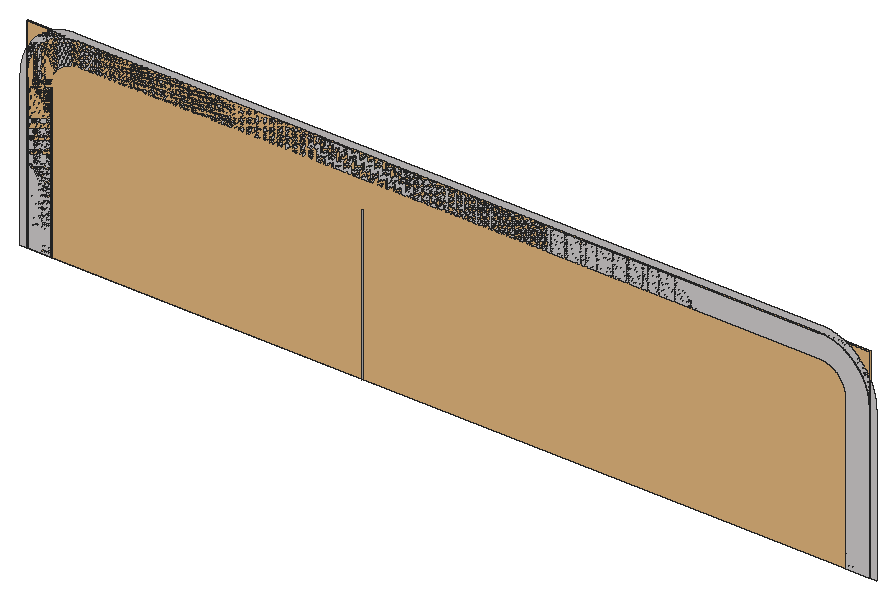
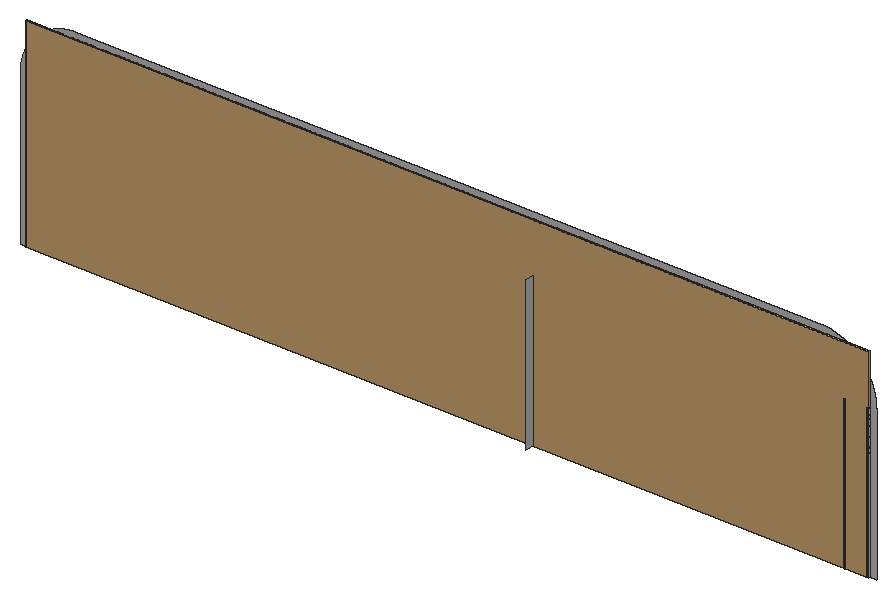
# SketchUp Ruby script. Lengths in inches.
U = 1.inch
M = Sketchup.active_model
def pt(a) = Geom::Point3d.new(a.map { |v| v * U })
def face(e, loops, mat)
  f = e.add_face(loops[0].map { |a| pt(a) })
  loops[1..].each { |l| e.add_face(l.map { |a| pt(a) }).erase! }
  f.material = f.back_material = mat if mat
  f
end
# faces: each face lists its corners as indices into pts; further lists are holes
def faces(e, pts, list, mat = nil) = list.each { |f| face(e, (f[0].is_a?(Array) ? f : [f]).map { |l| l.map { |i| pts[i] } }, mat) }
# xy, xz, yz: faces in a plane at the given z, y or x. An outline is a flat list of corners, or four numbers for a rectangle; further outlines are holes
def ring(l) = l.size == 4 ? [[l[0], l[1]], [l[2], l[1]], [l[2], l[3]], [l[0], l[3]]] : l.each_slice(2).to_a
def flat(e, list, mat, &to3) = list.each { |f| face(e, (f[0].is_a?(Array) ? f : [f]).map { |l| ring(l).map { |u, v| to3.(u, v) } }, mat) }
def xy(e, z, list, mat = nil) = flat(e, list, mat) { |x, y| [x, y, z] }
def xz(e, y, list, mat = nil) = flat(e, list, mat) { |x, z| [x, y, z] }
def yz(e, x, list, mat = nil) = flat(e, list, mat) { |y, z| [x, y, z] }
def lines(e, pts, list) = list.each { |a, b| e.add_line(pt(pts[a]), pt(pts[b])) }
# prism: a flat outline (further loops are holes) pulled along v
def prism(e, loops, v, mat = nil)
  f = face(e, loops, mat); d = Geom::Vector3d.new(v.map { |x| x * U })
  f.pushpull(f.normal.samedirection?(d) ? d.length : -d.length)
end
def box(e, o, s, mat = nil) = prism(e, [[o, [o[0] + s[0], o[1], o[2]], [o[0] + s[0], o[1] + s[1], o[2]], [o[0], o[1] + s[1], o[2]]]], [0, 0, s[2]], mat)
def at(x, y, z, deg = 0) = Geom::Transformation.translation(pt([x, y, z])) * Geom::Transformation.rotation(ORIGIN, Z_AXIS, deg.degrees)
def axes(o, x, y, z) = Geom::Transformation.new([*x, 0, *y, 0, *z, 0, *pt(o).to_a, 1])
def part(name) = M.definitions.add(name)
# library, detail: a bought-in or finely detailed component or shape, given as its bounding box
def library(name, o, s) = part(name).tap { |d| box(d.entities, o, s) }
def detail(e, o, s) = box(e.add_group.entities, o, s)
def put(e, d, t, mat = nil) = e.add_instance(d, t).tap { |i| i.material = mat if mat }
def group(e, t, mat = nil) = e.add_group.tap { |g| g.transformation = t; g.material = mat if mat }.entities
root = M.entities
M.materials.add("Outer Light - 1").color = [251, 216, 141]
M.materials.add("[Quartz Light Brown]").color = [215, 212, 212]
M.materials.add("[Stone Sandstone Ashlar Light]").color = [201, 199, 196]
c1 = library("Group\#55",[0,0,0],[532,1,128])
xz(root,38,[[0,-12,4,-12,4,84.5,4.01,84.75,4.02,85.01,4.02,85.26,4.04,85.51,4.05,85.76,4.0625,86.01,4.08,86.26,4.14,87.01,4.17,87.26,4.19,87.51,4.28,88.26,4.36,88.76,4.39,89.01,4.43,89.25,4.48,89.5,4.52,89.75,4.57,90,4.61,90.24,4.66,90.49,4.72,90.74,4.77,90.98,4.83,91.23,4.88,91.47,4.94,91.71,5.01,91.96,5.13,92.44,5.2,92.6875,5.27,92.93,5.41,93.41,5.57,93.89,5.64,94.13,5.73,94.37,5.81,94.6,5.89,94.84,5.98,95.08,6.07,95.3125,6.16,95.55,6.34,96.01,6.4375,96.25,6.53,96.48,6.63,96.71,6.73,96.9375,6.84,97.17,6.9375,97.4,7.05,97.625,7.15,97.85,7.26,98.08,7.375,98.3,7.6,98.75,7.72,98.97,7.84,99.2,8.08,99.64,8.2,99.85,8.59,100.51,8.85,100.93,8.98,101.15,9.12,101.36,9.25,101.57,9.53,101.99,9.68,102.19,9.96,102.61,10.41,103.21,10.5625,103.41,10.72,103.61,10.87,103.8125,11.03,104.01,11.18,104.2,11.34,104.4,11.5,104.59,11.67,104.78,11.83,104.97,12,105.16,12.16,105.35,12.33,105.54,12.5,105.72,12.67,105.91,12.85,106.09,13.02,106.27,13.2,106.45,13.37,106.63,13.55,106.8,13.73,106.98,13.91,107.15,14.09,107.33,14.28,107.5,14.46,107.67,14.65,107.84,14.84,108,15.03,108.17,15.22,108.33,15.41,108.5,15.6,108.66,15.8,108.82,15.99,108.97,16.1875,109.13,16.39,109.28,16.59,109.4375,16.79,109.59,17.39,110.04,17.81,110.32,18.01,110.47,18.43,110.75,18.64,110.88,18.85,111.02,19.07,111.15,19.49,111.41,20.15,111.8,20.36,111.92,20.8,112.16,21.03,112.28,21.25,112.4,21.7,112.625,21.92,112.74,22.15,112.85,22.375,112.95,22.6,113.0625,22.83,113.16,23.0625,113.27,23.29,113.37,23.52,113.47,23.75,113.5625,23.99,113.66,24.45,113.84,24.6875,113.93,24.92,114.02,25.16,114.11,25.4,114.19,25.63,114.27,25.87,114.36,26.11,114.43,26.59,114.59,27.07,114.73,27.3125,114.8,27.56,114.87,28.04,114.99,28.29,115.06,28.53,115.12,28.77,115.17,29.02,115.23,29.26,115.28,29.51,115.34,29.76,115.39,30,115.43,30.25,115.48,30.5,115.52,30.75,115.57,30.99,115.61,31.24,115.64,31.74,115.72,32.49,115.81,32.74,115.83,32.99,115.86,33.74,115.92,33.99,115.9375,34.24,115.95,34.49,115.96,34.74,115.98,34.99,115.98,35.25,115.99,35.5,116,504.5,116,504.75,115.99,505.01,115.98,505.26,115.98,505.51,115.96,505.76,115.95,506.01,115.9375,506.26,115.92,507.01,115.86,507.26,115.83,507.51,115.81,508.26,115.72,508.76,115.64,509.01,115.61,509.25,115.57,509.5,115.52,509.75,115.48,510,115.43,510.24,115.39,510.49,115.34,510.74,115.28,510.98,115.23,511.23,115.17,511.47,115.12,511.71,115.06,511.96,114.99,512.44,114.87,512.6875,114.8,512.93,114.73,513.41,114.59,513.89,114.43,514.13,114.36,514.37,114.27,514.6,114.19,514.84,114.11,515.08,114.02,515.3125,113.93,515.55,113.84,516.01,113.66,516.25,113.5625,516.48,113.47,516.71,113.37,516.9375,113.27,517.17,113.16,517.4,113.0625,517.625,112.95,517.85,112.85,518.08,112.74,518.3,112.625,518.75,112.4,518.97,112.28,519.2,112.16,519.64,111.92,519.85,111.8,520.51,111.41,520.93,111.15,521.15,111.02,521.36,110.88,521.57,110.75,521.99,110.47,522.19,110.32,522.61,110.04,523.21,109.59,523.41,109.4375,523.61,109.28,523.8125,109.13,524.01,108.97,524.2,108.82,524.4,108.66,524.59,108.5,524.78,108.33,524.97,108.17,525.16,108,525.35,107.84,525.54,107.67,525.72,107.5,525.91,107.33,526.09,107.15,526.27,106.98,526.45,106.8,526.63,106.63,526.8,106.45,526.98,106.27,527.15,106.09,527.33,105.91,527.5,105.72,527.67,105.54,527.84,105.35,528,105.16,528.17,104.97,528.33,104.78,528.5,104.59,528.66,104.4,528.82,104.2,528.97,104.01,529.13,103.8125,529.28,103.61,529.4375,103.41,529.59,103.21,530.04,102.61,530.32,102.19,530.47,101.99,530.75,101.57,530.88,101.36,531.02,101.15,531.15,100.93,531.41,100.51,531.8,99.85,531.92,99.64,532.16,99.2,532.28,98.97,532.4,98.75,532.625,98.3,532.74,98.08,532.85,97.85,532.95,97.625,533.0625,97.4,533.16,97.17,533.27,96.9375,533.37,96.71,533.47,96.48,533.5625,96.25,533.66,96.01,533.84,95.55,533.93,95.3125,534.02,95.08,534.11,94.84,534.19,94.6,534.27,94.37,534.36,94.13,534.43,93.89,534.59,93.41,534.73,92.93,534.8,92.6875,534.87,92.44,534.99,91.96,535.06,91.71,535.12,91.47,535.17,91.23,535.23,90.98,535.28,90.74,535.34,90.49,535.39,90.24,535.43,90,535.48,89.75,535.52,89.5,535.57,89.25,535.61,89.01,535.64,88.76,535.72,88.26,535.81,87.51,535.83,87.26,535.86,87.01,535.92,86.26,535.9375,86.01,535.95,85.76,535.96,85.51,535.98,85.26,535.98,85.01,535.99,84.75,536,84.5,536,-12,540,-12,540,84.57,539.97,85.41,539.96,85.7,539.95,85.98,539.89,86.82,539.87,87.11,539.84,87.39,539.8125,87.67,539.78,87.95,539.72,88.51,539.56,89.63,539.51,89.91,539.46,90.1875,539.41,90.47,539.36,90.75,539.31,91.02,539.19,91.58,539.13,91.85,539.07,92.13,539.01,92.4,538.9375,92.68,538.8,93.23,538.72,93.5,538.65,93.77,538.49,94.31,538.41,94.59,538.32,94.86,538.24,95.125,538.15,95.39,537.97,95.93,537.87,96.19,537.77,96.46,537.68,96.73,537.58,96.99,537.47,97.25,537.37,97.51,537.26,97.78,536.93,98.56,536.8125,98.81,536.69,99.07,536.57,99.33,536.45,99.58,536.33,99.84,536.2,100.09,536.08,100.34,535.95,100.6,535.82,100.85,535.68,101.09,535.55,101.34,535.27,101.84,535.13,102.08,534.99,102.33,534.84,102.57,534.7,102.81,534.4,103.29,534.24,103.53,534.09,103.76,533.77,104.24,533.62,104.47,533.45,104.7,533.29,104.93,532.96,105.39,532.79,105.62,532.45,106.06,532.27,106.29,532.1,106.51,531.74,106.95,531.56,107.16,531.375,107.38,531.19,107.59,531,107.81,530.82,108.02,530.625,108.23,530.4375,108.4375,530.24,108.64,530.05,108.85,529.85,109.05,529.65,109.26,529.46,109.46,529.26,109.65,529.05,109.85,528.85,110.05,528.64,110.24,528.4375,110.4375,528.23,110.625,528.02,110.82,527.81,111,527.59,111.19,527.38,111.375,527.16,111.56,526.95,111.74,526.51,112.1,526.29,112.27,526.06,112.45,525.62,112.79,525.39,112.96,524.93,113.29,524.7,113.45,524.47,113.62,524.24,113.77,523.76,114.09,523.53,114.24,523.29,114.4,522.81,114.7,522.57,114.84,522.33,114.99,522.08,115.13,521.84,115.27,521.34,115.55,521.09,115.68,520.85,115.82,520.6,115.95,520.34,116.08,520.09,116.2,519.84,116.33,519.58,116.45,519.33,116.57,519.07,116.69,518.81,116.8125,518.56,116.93,517.78,117.26,517.51,117.37,517.25,117.47,516.99,117.58,516.73,117.68,516.46,117.77,516.19,117.87,515.93,117.97,515.39,118.15,515.125,118.24,514.86,118.32,514.59,118.41,514.31,118.49,513.77,118.65,513.5,118.72,513.23,118.8,512.68,118.9375,512.4,119.01,512.13,119.07,511.85,119.13,511.58,119.19,511.02,119.31,510.75,119.36,510.47,119.41,510.1875,119.46,509.91,119.51,509.63,119.56,508.51,119.72,507.95,119.78,507.67,119.8125,507.39,119.84,507.11,119.87,506.82,119.89,505.98,119.95,505.7,119.96,505.41,119.97,504.57,120,35.43,120,34.59,119.97,34.3,119.96,34.02,119.95,33.18,119.89,32.89,119.87,32.61,119.84,32.33,119.8125,32.05,119.78,31.49,119.72,30.37,119.56,30.09,119.51,29.8125,119.46,29.53,119.41,29.25,119.36,28.98,119.31,28.42,119.19,28.15,119.13,27.87,119.07,27.6,119.01,27.32,118.9375,26.77,118.8,26.5,118.72,26.23,118.65,25.69,118.49,25.41,118.41,25.14,118.32,24.875,118.24,24.61,118.15,24.07,117.97,23.81,117.87,23.54,117.77,23.27,117.68,23.01,117.58,22.75,117.47,22.49,117.37,22.22,117.26,21.44,116.93,21.19,116.8125,20.93,116.69,20.67,116.57,20.42,116.45,20.16,116.33,19.91,116.2,19.66,116.08,19.4,115.95,19.15,115.82,18.91,115.68,18.66,115.55,18.16,115.27,17.92,115.13,17.67,114.99,17.43,114.84,17.19,114.7,16.71,114.4,16.47,114.24,16.24,114.09,15.76,113.77,15.53,113.62,15.3,113.45,15.07,113.29,14.61,112.96,14.38,112.79,13.94,112.45,13.71,112.27,13.49,112.1,13.05,111.74,12.84,111.56,12.62,111.375,12.41,111.19,12.19,111,11.98,110.82,11.77,110.625,11.5625,110.4375,11.36,110.24,11.15,110.05,10.95,109.85,10.74,109.65,10.54,109.46,10.35,109.26,10.15,109.05,9.95,108.85,9.76,108.64,9.5625,108.4375,9.375,108.23,9.18,108.02,9,107.81,8.81,107.59,8.625,107.38,8.44,107.16,8.26,106.95,7.9,106.51,7.73,106.29,7.55,106.06,7.21,105.62,7.04,105.39,6.71,104.93,6.55,104.7,6.38,104.47,6.23,104.24,5.91,103.76,5.76,103.53,5.6,103.29,5.3,102.81,5.16,102.57,5.01,102.33,4.87,102.08,4.73,101.84,4.45,101.34,4.32,101.09,4.18,100.85,4.05,100.6,3.92,100.34,3.8,100.09,3.67,99.84,3.55,99.58,3.43,99.33,3.31,99.07,3.1875,98.81,3.07,98.56,2.74,97.78,2.63,97.51,2.53,97.25,2.42,96.99,2.32,96.73,2.23,96.46,2.13,96.19,2.03,95.93,1.85,95.39,1.76,95.125,1.68,94.86,1.59,94.59,1.51,94.31,1.35,93.77,1.28,93.5,1.2,93.23,1.0625,92.68,0.99,92.4,0.93,92.13,0.87,91.85,0.81,91.58,0.69,91.02,0.64,90.75,0.59,90.47,0.54,90.1875,0.49,89.91,0.44,89.63,0.28,88.51,0.22,87.95,0.1875,87.67,0.16,87.39,0.13,87.11,0.11,86.82,0.05,85.98,0.04,85.7,0.03,85.41,0,84.57],[5,-12,19,-12,19,84.4,19.01,84.53,19.01,84.67,19.03,84.93,19.03,85.07,19.05,85.33,19.0625,85.47,19.08,85.6,19.09,85.73,19.1,85.87,19.12,86,19.13,86.13,19.15,86.26,19.17,86.4,19.1875,86.53,19.21,86.66,19.25,86.92,19.28,87.05,19.3,87.19,19.33,87.32,19.35,87.45,19.41,87.71,19.4375,87.84,19.47,87.97,19.53,88.23,19.57,88.36,19.6,88.49,19.64,88.61,19.68,88.74,19.71,88.87,19.75,89,19.83,89.25,19.92,89.51,19.96,89.63,20.01,89.76,20.05,89.88,20.1,90.01,20.15,90.13,20.19,90.26,20.24,90.38,20.29,90.51,20.35,90.63,20.4,90.75,20.45,90.875,20.51,91,20.5625,91.12,20.62,91.24,20.68,91.36,20.73,91.48,20.91,91.84,20.98,91.95,21.1,92.19,21.17,92.31,21.23,92.42,21.3,92.54,21.37,92.65,21.4375,92.77,21.51,92.88,21.58,93,21.79,93.33,21.87,93.44,21.94,93.56,22.02,93.67,22.09,93.78,22.17,93.88,22.41,94.21,22.49,94.3125,22.57,94.42,22.65,94.52,22.73,94.63,22.82,94.73,22.9,94.84,22.99,94.9375,23.07,95.04,23.61,95.64,23.7,95.73,23.79,95.83,24.17,96.21,24.27,96.3,24.36,96.39,24.96,96.93,25.0625,97.01,25.16,97.1,25.27,97.18,25.37,97.27,25.48,97.35,25.58,97.43,25.6875,97.51,25.79,97.59,26.12,97.83,26.22,97.91,26.33,97.98,26.44,98.06,26.56,98.13,26.67,98.21,27,98.42,27.12,98.49,27.23,98.5625,27.35,98.63,27.46,98.7,27.58,98.77,27.69,98.83,27.81,98.9,28.05,99.02,28.16,99.09,28.52,99.27,28.64,99.32,28.76,99.38,28.88,99.4375,29,99.49,29.125,99.55,29.25,99.6,29.37,99.65,29.49,99.71,29.62,99.76,29.74,99.81,29.87,99.85,29.99,99.9,30.12,99.95,30.24,99.99,30.37,100.04,30.49,100.08,30.75,100.17,31,100.25,31.13,100.29,31.26,100.32,31.39,100.36,31.51,100.4,31.64,100.43,31.77,100.47,32.03,100.53,32.16,100.5625,32.29,100.59,32.55,100.65,32.68,100.67,32.81,100.7,32.95,100.72,33.08,100.75,33.34,100.79,33.47,100.8125,33.6,100.83,33.74,100.85,33.87,100.87,34,100.88,34.13,100.9,34.27,100.91,34.4,100.92,34.53,100.9375,34.67,100.95,34.93,100.97,35.07,100.97,35.33,100.99,35.47,100.99,35.6,101,504.4,101,504.53,100.99,504.67,100.99,504.93,100.97,505.07,100.97,505.33,100.95,505.47,100.9375,505.6,100.92,505.73,100.91,505.87,100.9,506,100.88,506.13,100.87,506.26,100.85,506.4,100.83,506.53,100.8125,506.66,100.79,506.92,100.75,507.05,100.72,507.19,100.7,507.32,100.67,507.45,100.65,507.71,100.59,507.84,100.5625,507.97,100.53,508.23,100.47,508.36,100.43,508.49,100.4,508.61,100.36,508.74,100.32,508.87,100.29,509,100.25,509.25,100.17,509.51,100.08,509.63,100.04,509.76,99.99,509.88,99.95,510.01,99.9,510.13,99.85,510.26,99.81,510.38,99.76,510.51,99.71,510.63,99.65,510.75,99.6,510.875,99.55,511,99.49,511.12,99.4375,511.24,99.38,511.36,99.32,511.48,99.27,511.84,99.09,511.95,99.02,512.19,98.9,512.31,98.83,512.42,98.77,512.54,98.7,512.65,98.63,512.77,98.5625,512.88,98.49,513,98.42,513.33,98.21,513.44,98.13,513.56,98.06,513.67,97.98,513.78,97.91,513.88,97.83,514.21,97.59,514.3125,97.51,514.42,97.43,514.52,97.35,514.63,97.27,514.73,97.18,514.84,97.1,514.9375,97.01,515.04,96.93,515.64,96.39,515.73,96.3,515.83,96.21,516.21,95.83,516.3,95.73,516.39,95.64,516.93,95.04,517.01,94.9375,517.1,94.84,517.18,94.73,517.27,94.63,517.35,94.52,517.43,94.42,517.51,94.3125,517.59,94.21,517.83,93.88,517.91,93.78,517.98,93.67,518.06,93.56,518.13,93.44,518.21,93.33,518.42,93,518.49,92.88,518.5625,92.77,518.63,92.65,518.7,92.54,518.77,92.42,518.83,92.31,518.9,92.19,519.02,91.95,519.09,91.84,519.27,91.48,519.32,91.36,519.38,91.24,519.4375,91.12,519.49,91,519.55,90.875,519.6,90.75,519.65,90.63,519.71,90.51,519.76,90.38,519.81,90.26,519.85,90.13,519.9,90.01,519.95,89.88,519.99,89.76,520.04,89.63,520.08,89.51,520.17,89.25,520.25,89,520.29,88.87,520.32,88.74,520.36,88.61,520.4,88.49,520.43,88.36,520.47,88.23,520.53,87.97,520.5625,87.84,520.59,87.71,520.65,87.45,520.67,87.32,520.7,87.19,520.72,87.05,520.75,86.92,520.79,86.66,520.8125,86.53,520.83,86.4,520.85,86.26,520.87,86.13,520.88,86,520.9,85.87,520.91,85.73,520.92,85.6,520.9375,85.47,520.95,85.33,520.97,85.07,520.97,84.93,520.99,84.67,520.99,84.53,521,84.4,521,-12,535,-12,535,84.49,534.98,84.97,534.98,85.22,534.97,85.46,534.95,85.7,534.9375,85.95,534.92,86.1875,534.9,86.43,534.88,86.67,534.86,86.92,534.84,87.16,534.8125,87.4,534.79,87.64,534.76,87.89,534.72,88.125,534.69,88.37,534.66,88.61,534.5,89.57,534.4,90.05,534.36,90.29,534.31,90.52,534.25,90.76,534.2,91,534.14,91.24,534.09,91.47,534.03,91.71,533.96,91.94,533.9,92.18,533.84,92.41,533.77,92.65,533.7,92.88,533.63,93.12,533.56,93.35,533.48,93.58,533.41,93.8125,533.33,94.04,533.17,94.5,533.08,94.73,533,94.96,532.91,95.19,532.82,95.41,532.73,95.64,532.64,95.86,532.55,96.09,532.45,96.3125,532.35,96.53,532.25,96.76,531.95,97.42,531.73,97.86,531.62,98.07,531.4,98.51,531.28,98.72,531.17,98.93,531.05,99.15,530.81,99.57,530.68,99.78,530.56,99.99,530.43,100.2,530.3,100.4,530.04,100.82,529.78,101.22,529.64,101.42,529.36,101.83,529.22,102.02,529.08,102.22,528.9375,102.42,528.79,102.61,528.64,102.81,527.89,103.76,527.73,103.95,527.57,104.13,527.41,104.32,526.93,104.86,526.76,105.04,526.6,105.22,526.43,105.4,526.26,105.57,526.09,105.75,525.75,106.09,525.57,106.26,525.4,106.43,525.22,106.6,525.04,106.76,524.86,106.93,524.32,107.41,524.13,107.57,523.95,107.73,523.76,107.89,522.81,108.64,522.61,108.79,522.42,108.9375,522.22,109.08,522.02,109.22,521.83,109.36,521.42,109.64,521.22,109.78,520.82,110.04,520.4,110.3,520.2,110.43,519.99,110.56,519.78,110.68,519.57,110.81,519.15,111.05,518.93,111.17,518.72,111.28,518.51,111.4,518.07,111.62,517.86,111.73,517.42,111.95,516.76,112.25,516.53,112.35,516.3125,112.45,516.09,112.55,515.86,112.64,515.64,112.73,515.41,112.82,515.19,112.91,514.96,113,514.73,113.08,514.5,113.17,514.04,113.33,513.8125,113.41,513.58,113.48,513.35,113.56,513.12,113.63,512.88,113.7,512.65,113.77,512.41,113.84,512.18,113.9,511.94,113.96,511.71,114.03,511.47,114.09,511.24,114.14,511,114.2,510.76,114.25,510.52,114.31,510.29,114.36,510.05,114.4,509.57,114.5,508.61,114.66,508.37,114.69,508.125,114.72,507.89,114.76,507.64,114.79,507.4,114.8125,507.16,114.84,506.92,114.86,506.67,114.88,506.43,114.9,506.1875,114.92,505.95,114.9375,505.7,114.95,505.46,114.97,505.22,114.98,504.97,114.98,504.49,115,35.51,115,35.03,114.98,34.78,114.98,34.54,114.97,34.3,114.95,34.05,114.9375,33.8125,114.92,33.57,114.9,33.33,114.88,33.08,114.86,32.84,114.84,32.6,114.8125,32.36,114.79,32.11,114.76,31.875,114.72,31.63,114.69,31.39,114.66,30.43,114.5,29.95,114.4,29.71,114.36,29.48,114.31,29.24,114.25,29,114.2,28.76,114.14,28.53,114.09,28.29,114.03,28.06,113.96,27.82,113.9,27.59,113.84,27.35,113.77,27.12,113.7,26.88,113.63,26.65,113.56,26.42,113.48,26.1875,113.41,25.96,113.33,25.5,113.17,25.27,113.08,25.04,113,24.81,112.91,24.59,112.82,24.36,112.73,24.14,112.64,23.91,112.55,23.6875,112.45,23.47,112.35,23.24,112.25,22.58,111.95,22.14,111.73,21.93,111.62,21.49,111.4,21.28,111.28,21.07,111.17,20.85,111.05,20.43,110.81,20.22,110.68,20.01,110.56,19.8,110.43,19.6,110.3,19.18,110.04,18.78,109.78,18.58,109.64,18.17,109.36,17.98,109.22,17.78,109.08,17.58,108.9375,17.39,108.79,17.19,108.64,16.24,107.89,16.05,107.73,15.87,107.57,15.68,107.41,15.14,106.93,14.96,106.76,14.78,106.6,14.6,106.43,14.43,106.26,14.25,106.09,13.91,105.75,13.74,105.57,13.57,105.4,13.4,105.22,13.24,105.04,13.07,104.86,12.59,104.32,12.43,104.13,12.27,103.95,12.11,103.76,11.36,102.81,11.21,102.61,11.0625,102.42,10.92,102.22,10.78,102.02,10.64,101.83,10.36,101.42,10.22,101.22,9.96,100.82,9.7,100.4,9.57,100.2,9.44,99.99,9.32,99.78,9.19,99.57,8.95,99.15,8.83,98.93,8.72,98.72,8.6,98.51,8.38,98.07,8.27,97.86,8.05,97.42,7.75,96.76,7.65,96.53,7.55,96.3125,7.45,96.09,7.36,95.86,7.27,95.64,7.18,95.41,7.09,95.19,7,94.96,6.92,94.73,6.83,94.5,6.67,94.04,6.59,93.8125,6.52,93.58,6.44,93.35,6.37,93.12,6.3,92.88,6.23,92.65,6.16,92.41,6.1,92.18,6.04,91.94,5.97,91.71,5.91,91.47,5.86,91.24,5.8,91,5.75,90.76,5.69,90.52,5.64,90.29,5.6,90.05,5.5,89.57,5.34,88.61,5.31,88.37,5.28,88.125,5.24,87.89,5.21,87.64,5.1875,87.4,5.16,87.16,5.14,86.92,5.12,86.67,5.1,86.43,5.08,86.1875,5.0625,85.95,5.05,85.7,5.03,85.46,5.02,85.22,5.02,84.97,5,84.49]],"[Quartz Light Brown]")
yz(root,4,[[38,-12,39,83.99]],"[Quartz Light Brown]")
yz(root,5,[[38,-12,39,83.99]],"[Quartz Light Brown]")
yz(root,19,[[38,-12,39,83.96]],"[Quartz Light Brown]")
yz(root,20,[[38,-12,39,83.96]],"[Quartz Light Brown]")
yz(root,216,[[37,-12,44,84]],"[Stone Sandstone Ashlar Light]")
put(root,c1,at(4,38,-12),"Outer Light - 1")
